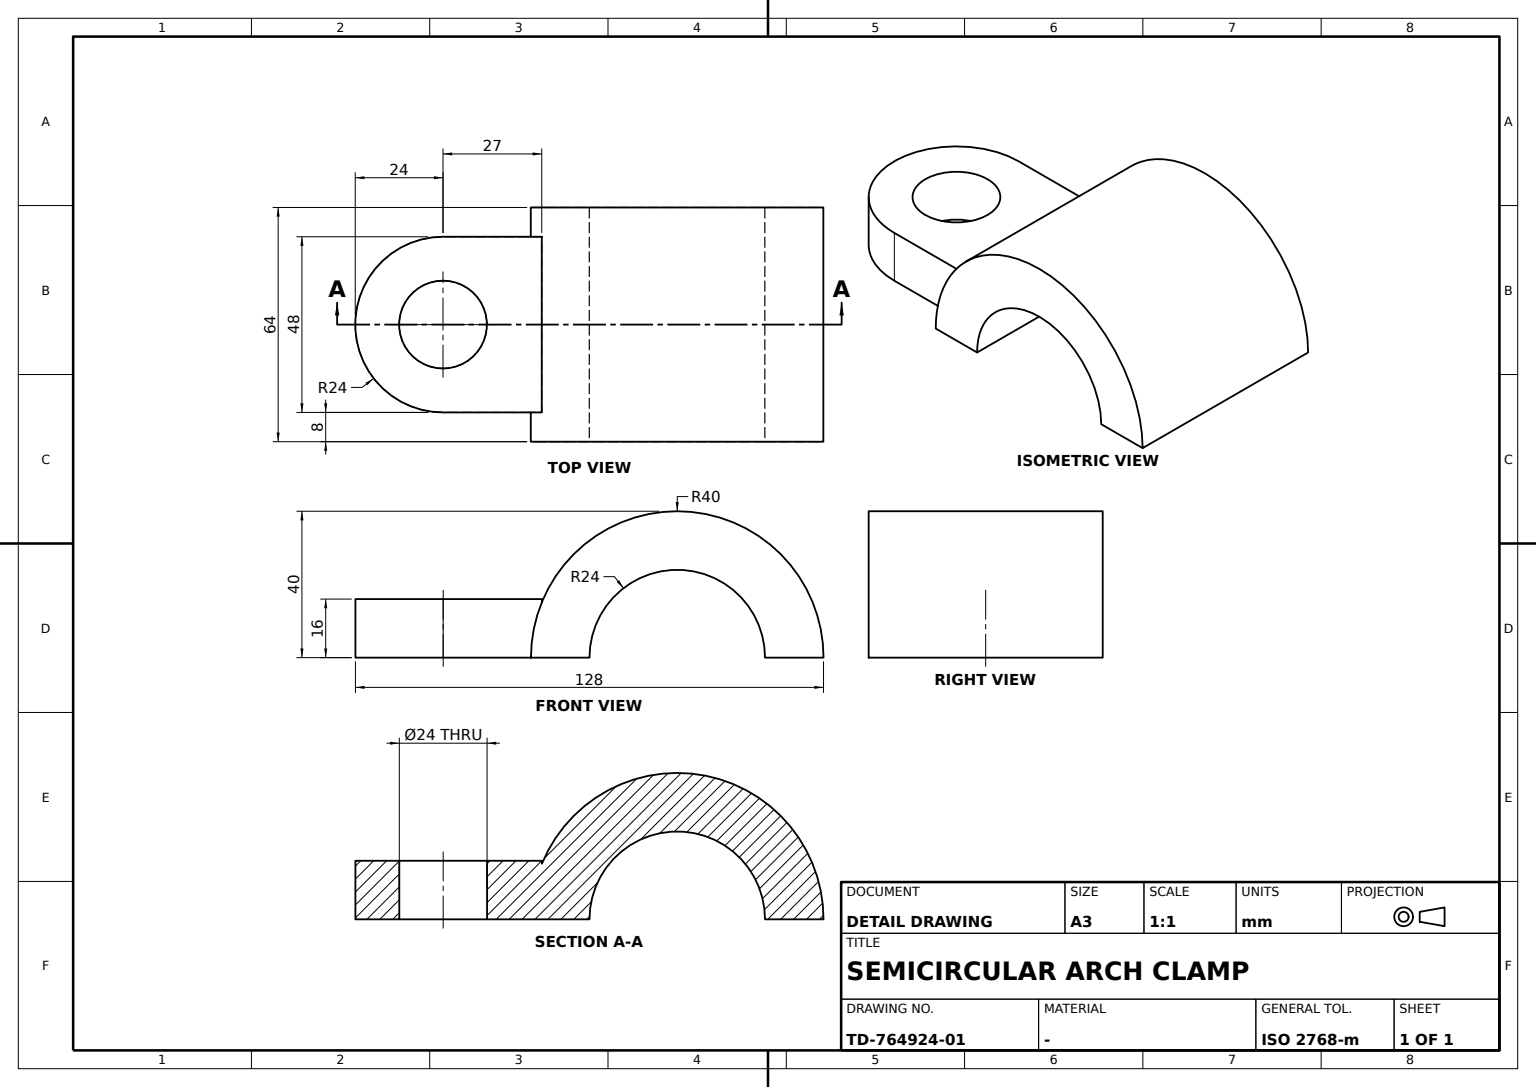
ISO-10303-21;
HEADER;
FILE_DESCRIPTION((''),'2;1');
FILE_NAME('','',(''),(''),'','','');
FILE_SCHEMA(('AUTOMOTIVE_DESIGN'));
ENDSEC;
DATA;
#1=APPLICATION_CONTEXT('');
#2=PRODUCT_CONTEXT('',#1,'mechanical');
#3=PRODUCT('','','',(#2));
#4=PRODUCT_DEFINITION_FORMATION('','',#3);
#5=PRODUCT_DEFINITION_CONTEXT('',#1,'design');
#6=PRODUCT_DEFINITION('','',#4,#5);
#7=PRODUCT_DEFINITION_SHAPE('','',#6);
#8=(LENGTH_UNIT()NAMED_UNIT(*)SI_UNIT(.MILLI.,.METRE.));
#9=(NAMED_UNIT(*)PLANE_ANGLE_UNIT()SI_UNIT($,.RADIAN.));
#10=(NAMED_UNIT(*)SI_UNIT($,.STERADIAN.)SOLID_ANGLE_UNIT());
#11=UNCERTAINTY_MEASURE_WITH_UNIT(LENGTH_MEASURE(0.005),#8,'distance_accuracy_value','');
#12=(GEOMETRIC_REPRESENTATION_CONTEXT(3)GLOBAL_UNCERTAINTY_ASSIGNED_CONTEXT((#11))GLOBAL_UNIT_ASSIGNED_CONTEXT((#8,#9,#10))REPRESENTATION_CONTEXT('',''));
#13=CARTESIAN_POINT('',(12.,-64.,16.));
#14=VERTEX_POINT('',#13);
#15=CARTESIAN_POINT('',(0.,-64.,16.));
#16=DIRECTION('',(0.,0.,1.));
#17=DIRECTION('',(1.,0.,0.));
#18=AXIS2_PLACEMENT_3D('',#15,#16,#17);
#19=CIRCLE('',#18,12.);
#20=EDGE_CURVE('',#14,#14,#19,.T.);
#21=ORIENTED_EDGE('',*,*,#20,.F.);
#22=EDGE_LOOP('',(#21));
#23=FACE_BOUND('',#22,.T.);
#24=CARTESIAN_POINT('',(24.,-37.,16.));
#25=VERTEX_POINT('',#24);
#26=CARTESIAN_POINT('',(24.,-64.,16.));
#27=VERTEX_POINT('',#26);
#28=CARTESIAN_POINT('',(24.,0.,16.));
#29=DIRECTION('',(0.,-1.,0.));
#30=VECTOR('',#29,1000.);
#31=LINE('',#28,#30);
#32=EDGE_CURVE('',#25,#27,#31,.T.);
#33=ORIENTED_EDGE('',*,*,#32,.F.);
#34=CARTESIAN_POINT('',(-24.,-37.,16.));
#35=VERTEX_POINT('',#34);
#36=CARTESIAN_POINT('',(0.,-37.,16.));
#37=VECTOR('',#17,1000.);
#38=LINE('',#36,#37);
#39=EDGE_CURVE('',#35,#25,#38,.T.);
#40=ORIENTED_EDGE('',*,*,#39,.F.);
#41=CARTESIAN_POINT('',(-24.,-64.,16.));
#42=VERTEX_POINT('',#41);
#43=CARTESIAN_POINT('',(-24.,0.,16.));
#44=DIRECTION('',(0.,1.,0.));
#45=VECTOR('',#44,1000.);
#46=LINE('',#43,#45);
#47=EDGE_CURVE('',#42,#35,#46,.T.);
#48=ORIENTED_EDGE('',*,*,#47,.F.);
#49=CIRCLE('',#18,24.);
#50=EDGE_CURVE('',#42,#27,#49,.T.);
#51=ORIENTED_EDGE('',*,*,#50,.T.);
#52=EDGE_LOOP('',(#33,#40,#48,#51));
#53=FACE_BOUND('',#52,.T.);
#54=CARTESIAN_POINT('',(0.,0.,16.));
#55=AXIS2_PLACEMENT_3D('',#54,#16,#17);
#56=PLANE('',#55);
#57=ADVANCED_FACE('',(#23,#53),#56,.T.);
#58=CARTESIAN_POINT('',(-24.,-37.,15.198684));
#59=VERTEX_POINT('',#58);
#60=CARTESIAN_POINT('',(-24.,-37.,0.));
#61=VECTOR('',#16,1000.);
#62=LINE('',#60,#61);
#63=EDGE_CURVE('',#59,#35,#62,.T.);
#64=ORIENTED_EDGE('',*,*,#63,.T.);
#65=ORIENTED_EDGE('',*,*,#39,.T.);
#66=CARTESIAN_POINT('',(24.,-37.,15.198684));
#67=VERTEX_POINT('',#66);
#68=CARTESIAN_POINT('',(24.,-37.,0.));
#69=LINE('',#68,#61);
#70=EDGE_CURVE('',#67,#25,#69,.T.);
#71=ORIENTED_EDGE('',*,*,#70,.F.);
#72=LINE('',#58,#37);
#73=EDGE_CURVE('',#59,#67,#72,.T.);
#74=ORIENTED_EDGE('',*,*,#73,.F.);
#75=EDGE_LOOP('',(#64,#65,#71,#74));
#76=FACE_BOUND('',#75,.T.);
#77=AXIS2_PLACEMENT_3D('',#60,#29,#17);
#78=PLANE('',#77);
#79=ADVANCED_FACE('',(#76),#78,.F.);
#80=CARTESIAN_POINT('',(-12.,-64.,0.));
#81=VERTEX_POINT('',#80);
#82=CARTESIAN_POINT('',(0.,-64.,0.));
#83=DIRECTION('',(0.,0.,-1.));
#84=DIRECTION('',(-1.,0.,0.));
#85=AXIS2_PLACEMENT_3D('',#82,#83,#84);
#86=CIRCLE('',#85,12.);
#87=EDGE_CURVE('',#81,#81,#86,.F.);
#88=ORIENTED_EDGE('',*,*,#87,.F.);
#89=EDGE_LOOP('',(#88));
#90=FACE_BOUND('',#89,.T.);
#91=ORIENTED_EDGE('',*,*,#20,.T.);
#92=EDGE_LOOP('',(#91));
#93=FACE_BOUND('',#92,.T.);
#94=CARTESIAN_POINT('',(0.,-64.,8.));
#95=AXIS2_PLACEMENT_3D('',#94,#16,#17);
#96=CYLINDRICAL_SURFACE('',#95,12.);
#97=ADVANCED_FACE('',(#90,#93),#96,.F.);
#98=CARTESIAN_POINT('',(24.,-40.,0.));
#99=VERTEX_POINT('',#98);
#100=CARTESIAN_POINT('',(24.,-64.,0.));
#101=VERTEX_POINT('',#100);
#102=LINE('',#68,#30);
#103=EDGE_CURVE('',#99,#101,#102,.T.);
#104=ORIENTED_EDGE('',*,*,#103,.F.);
#105=CARTESIAN_POINT('',(24.,0.,0.));
#106=AXIS2_PLACEMENT_3D('',#105,#84,#16);
#107=CIRCLE('',#106,40.);
#108=EDGE_CURVE('',#99,#67,#107,.T.);
#109=ORIENTED_EDGE('',*,*,#108,.T.);
#110=ORIENTED_EDGE('',*,*,#70,.T.);
#111=ORIENTED_EDGE('',*,*,#32,.T.);
#112=CARTESIAN_POINT('',(24.,-64.,8.));
#113=LINE('',#112,#61);
#114=EDGE_CURVE('',#101,#27,#113,.T.);
#115=ORIENTED_EDGE('',*,*,#114,.F.);
#116=EDGE_LOOP('',(#104,#109,#110,#111,#115));
#117=FACE_BOUND('',#116,.T.);
#118=AXIS2_PLACEMENT_3D('',#68,#84,#29);
#119=PLANE('',#118);
#120=ADVANCED_FACE('',(#117),#119,.F.);
#121=CARTESIAN_POINT('',(-24.,-64.,0.));
#122=VERTEX_POINT('',#121);
#123=CARTESIAN_POINT('',(-24.,-64.,8.));
#124=LINE('',#123,#61);
#125=EDGE_CURVE('',#122,#42,#124,.T.);
#126=ORIENTED_EDGE('',*,*,#125,.T.);
#127=ORIENTED_EDGE('',*,*,#47,.T.);
#128=ORIENTED_EDGE('',*,*,#63,.F.);
#129=CARTESIAN_POINT('',(-24.,-40.,0.));
#130=VERTEX_POINT('',#129);
#131=CARTESIAN_POINT('',(-24.,0.,0.));
#132=AXIS2_PLACEMENT_3D('',#131,#17,#83);
#133=CIRCLE('',#132,40.);
#134=EDGE_CURVE('',#59,#130,#133,.T.);
#135=ORIENTED_EDGE('',*,*,#134,.T.);
#136=LINE('',#121,#45);
#137=EDGE_CURVE('',#122,#130,#136,.T.);
#138=ORIENTED_EDGE('',*,*,#137,.F.);
#139=EDGE_LOOP('',(#126,#127,#128,#135,#138));
#140=FACE_BOUND('',#139,.T.);
#141=AXIS2_PLACEMENT_3D('',#121,#17,#44);
#142=PLANE('',#141);
#143=ADVANCED_FACE('',(#140),#142,.F.);
#144=CARTESIAN_POINT('',(-32.,40.,0.));
#145=VERTEX_POINT('',#144);
#146=CARTESIAN_POINT('',(32.,40.,0.));
#147=VERTEX_POINT('',#146);
#148=LINE('',#144,#37);
#149=EDGE_CURVE('',#145,#147,#148,.T.);
#150=ORIENTED_EDGE('',*,*,#149,.F.);
#151=CARTESIAN_POINT('',(-32.,-40.,0.));
#152=VERTEX_POINT('',#151);
#153=CARTESIAN_POINT('',(-32.,0.,0.));
#154=AXIS2_PLACEMENT_3D('',#153,#17,#83);
#155=CIRCLE('',#154,40.);
#156=EDGE_CURVE('',#145,#152,#155,.T.);
#157=ORIENTED_EDGE('',*,*,#156,.T.);
#158=LINE('',#151,#37);
#159=EDGE_CURVE('',#152,#130,#158,.T.);
#160=ORIENTED_EDGE('',*,*,#159,.T.);
#161=ORIENTED_EDGE('',*,*,#134,.F.);
#162=ORIENTED_EDGE('',*,*,#73,.T.);
#163=ORIENTED_EDGE('',*,*,#108,.F.);
#164=CARTESIAN_POINT('',(32.,-40.,0.));
#165=VERTEX_POINT('',#164);
#166=LINE('',#98,#37);
#167=EDGE_CURVE('',#99,#165,#166,.T.);
#168=ORIENTED_EDGE('',*,*,#167,.T.);
#169=CARTESIAN_POINT('',(32.,0.,0.));
#170=AXIS2_PLACEMENT_3D('',#169,#17,#83);
#171=CIRCLE('',#170,40.);
#172=EDGE_CURVE('',#147,#165,#171,.T.);
#173=ORIENTED_EDGE('',*,*,#172,.F.);
#174=EDGE_LOOP('',(#150,#157,#160,#161,#162,#163,#168,#173));
#175=FACE_BOUND('',#174,.T.);
#176=CARTESIAN_POINT('',(0.,0.,0.));
#177=AXIS2_PLACEMENT_3D('',#176,#17,#44);
#178=CYLINDRICAL_SURFACE('',#177,40.);
#179=ADVANCED_FACE('',(#175),#178,.T.);
#180=CARTESIAN_POINT('',(32.,24.,0.));
#181=VERTEX_POINT('',#180);
#182=CARTESIAN_POINT('',(32.,-24.,0.));
#183=VERTEX_POINT('',#182);
#184=CIRCLE('',#170,24.);
#185=EDGE_CURVE('',#181,#183,#184,.T.);
#186=ORIENTED_EDGE('',*,*,#185,.T.);
#187=CARTESIAN_POINT('',(-32.,-24.,0.));
#188=VERTEX_POINT('',#187);
#189=LINE('',#187,#37);
#190=EDGE_CURVE('',#188,#183,#189,.T.);
#191=ORIENTED_EDGE('',*,*,#190,.F.);
#192=CARTESIAN_POINT('',(-32.,24.,0.));
#193=VERTEX_POINT('',#192);
#194=CIRCLE('',#154,24.);
#195=EDGE_CURVE('',#193,#188,#194,.T.);
#196=ORIENTED_EDGE('',*,*,#195,.F.);
#197=LINE('',#192,#37);
#198=EDGE_CURVE('',#193,#181,#197,.T.);
#199=ORIENTED_EDGE('',*,*,#198,.T.);
#200=EDGE_LOOP('',(#186,#191,#196,#199));
#201=FACE_BOUND('',#200,.T.);
#202=CYLINDRICAL_SURFACE('',#177,24.);
#203=ADVANCED_FACE('',(#201),#202,.F.);
#204=LINE('',#153,#45);
#205=EDGE_CURVE('',#193,#145,#204,.T.);
#206=ORIENTED_EDGE('',*,*,#205,.T.);
#207=ORIENTED_EDGE('',*,*,#149,.T.);
#208=LINE('',#169,#45);
#209=EDGE_CURVE('',#181,#147,#208,.T.);
#210=ORIENTED_EDGE('',*,*,#209,.F.);
#211=ORIENTED_EDGE('',*,*,#198,.F.);
#212=EDGE_LOOP('',(#206,#207,#210,#211));
#213=FACE_BOUND('',#212,.T.);
#214=CARTESIAN_POINT('',(0.,-40.,0.));
#215=AXIS2_PLACEMENT_3D('',#214,#83,#44);
#216=PLANE('',#215);
#217=ADVANCED_FACE('',(#213),#216,.T.);
#218=ORIENTED_EDGE('',*,*,#195,.T.);
#219=EDGE_CURVE('',#152,#188,#204,.T.);
#220=ORIENTED_EDGE('',*,*,#219,.F.);
#221=ORIENTED_EDGE('',*,*,#156,.F.);
#222=ORIENTED_EDGE('',*,*,#205,.F.);
#223=EDGE_LOOP('',(#218,#220,#221,#222));
#224=FACE_BOUND('',#223,.T.);
#225=AXIS2_PLACEMENT_3D('',#153,#17,#44);
#226=PLANE('',#225);
#227=ADVANCED_FACE('',(#224),#226,.F.);
#228=ORIENTED_EDGE('',*,*,#172,.T.);
#229=EDGE_CURVE('',#165,#183,#208,.T.);
#230=ORIENTED_EDGE('',*,*,#229,.T.);
#231=ORIENTED_EDGE('',*,*,#185,.F.);
#232=ORIENTED_EDGE('',*,*,#209,.T.);
#233=EDGE_LOOP('',(#228,#230,#231,#232));
#234=FACE_BOUND('',#233,.T.);
#235=AXIS2_PLACEMENT_3D('',#169,#17,#44);
#236=PLANE('',#235);
#237=ADVANCED_FACE('',(#234),#236,.T.);
#238=ORIENTED_EDGE('',*,*,#159,.F.);
#239=ORIENTED_EDGE('',*,*,#219,.T.);
#240=ORIENTED_EDGE('',*,*,#190,.T.);
#241=ORIENTED_EDGE('',*,*,#229,.F.);
#242=ORIENTED_EDGE('',*,*,#167,.F.);
#243=ORIENTED_EDGE('',*,*,#103,.T.);
#244=CIRCLE('',#85,24.);
#245=EDGE_CURVE('',#122,#101,#244,.F.);
#246=ORIENTED_EDGE('',*,*,#245,.F.);
#247=ORIENTED_EDGE('',*,*,#137,.T.);
#248=EDGE_LOOP('',(#238,#239,#240,#241,#242,#243,#246,#247));
#249=FACE_BOUND('',#248,.T.);
#250=ORIENTED_EDGE('',*,*,#87,.T.);
#251=EDGE_LOOP('',(#250));
#252=FACE_BOUND('',#251,.T.);
#253=ADVANCED_FACE('',(#249,#252),#216,.T.);
#254=ORIENTED_EDGE('',*,*,#50,.F.);
#255=ORIENTED_EDGE('',*,*,#125,.F.);
#256=ORIENTED_EDGE('',*,*,#245,.T.);
#257=ORIENTED_EDGE('',*,*,#114,.T.);
#258=EDGE_LOOP('',(#254,#255,#256,#257));
#259=FACE_BOUND('',#258,.T.);
#260=CYLINDRICAL_SURFACE('',#95,24.);
#261=ADVANCED_FACE('',(#259),#260,.T.);
#262=CLOSED_SHELL('',(#57,#79,#97,#120,#143,#179,#203,#217,#227,#237,#253,#261));
#263=MANIFOLD_SOLID_BREP('',#262);
#264=ADVANCED_BREP_SHAPE_REPRESENTATION('',(#263),#12);
#265=SHAPE_DEFINITION_REPRESENTATION(#7,#264);
ENDSEC;
END-ISO-10303-21;
